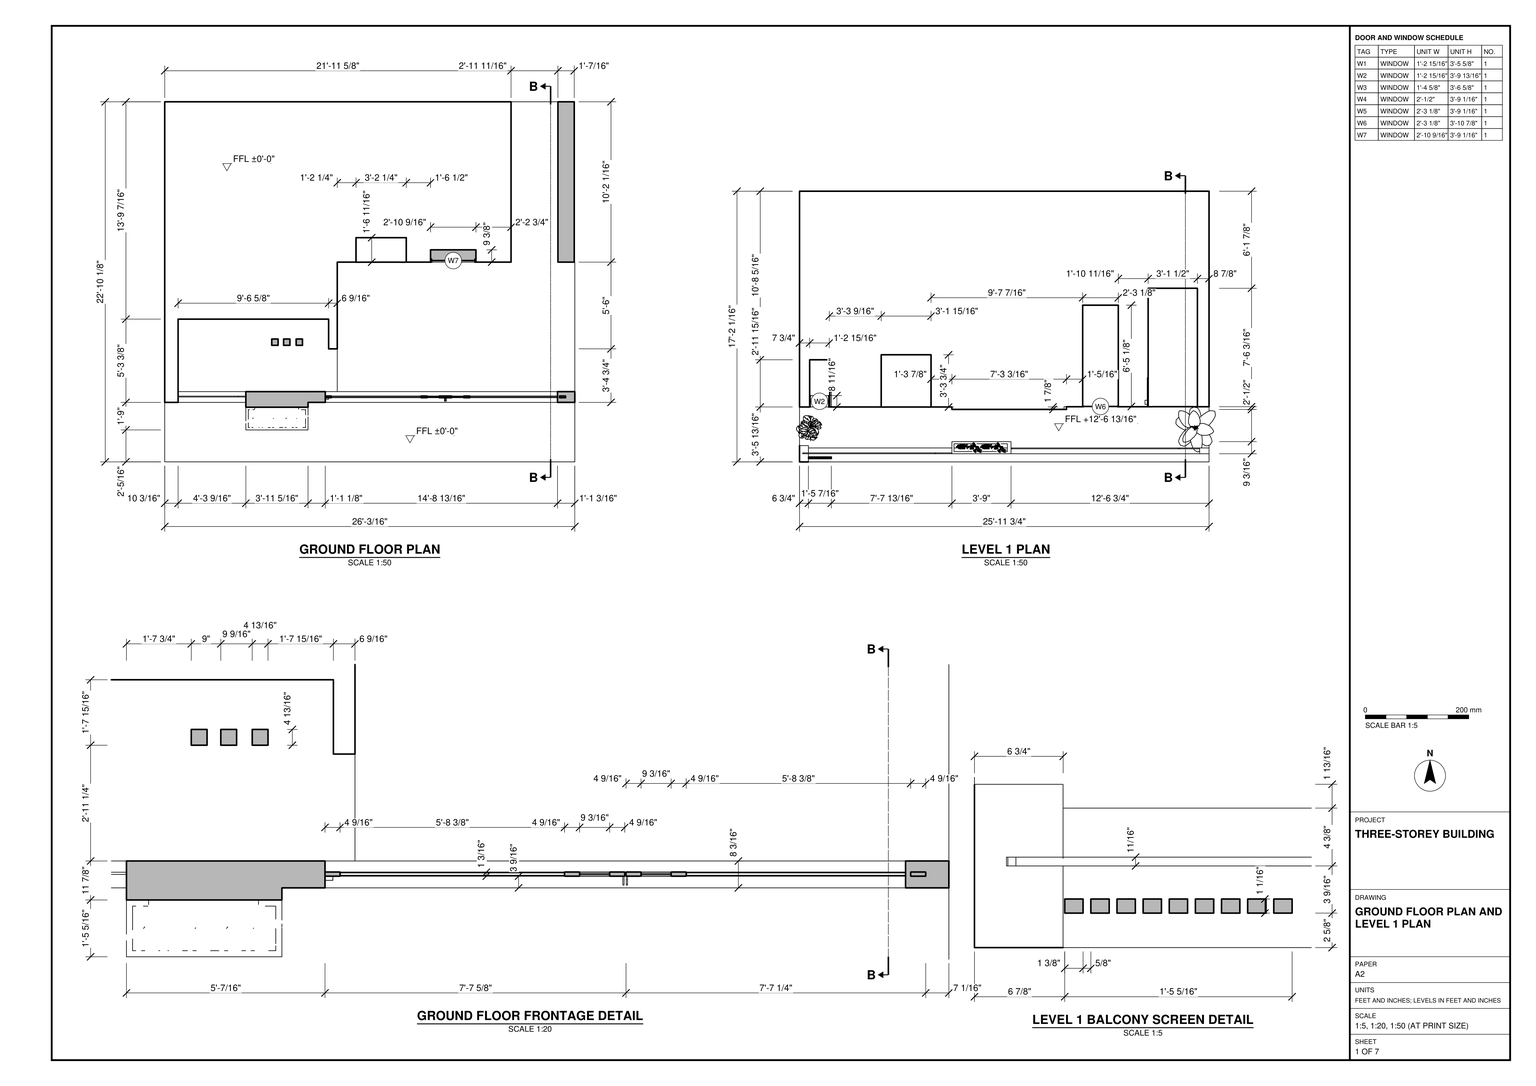
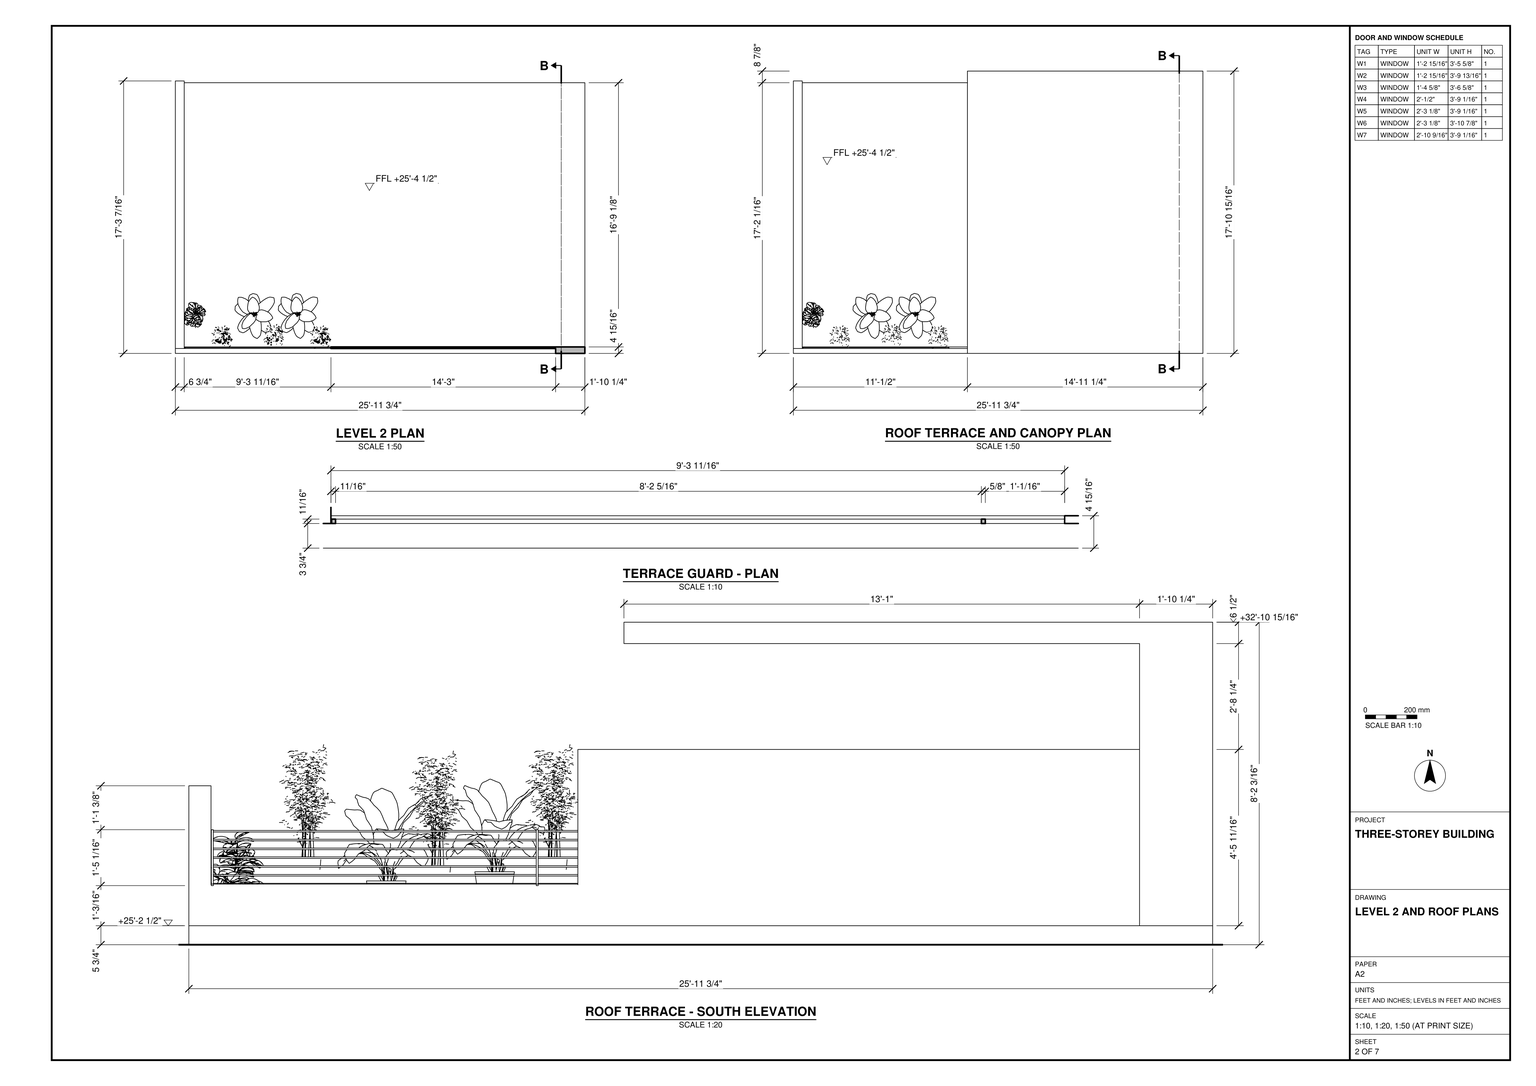
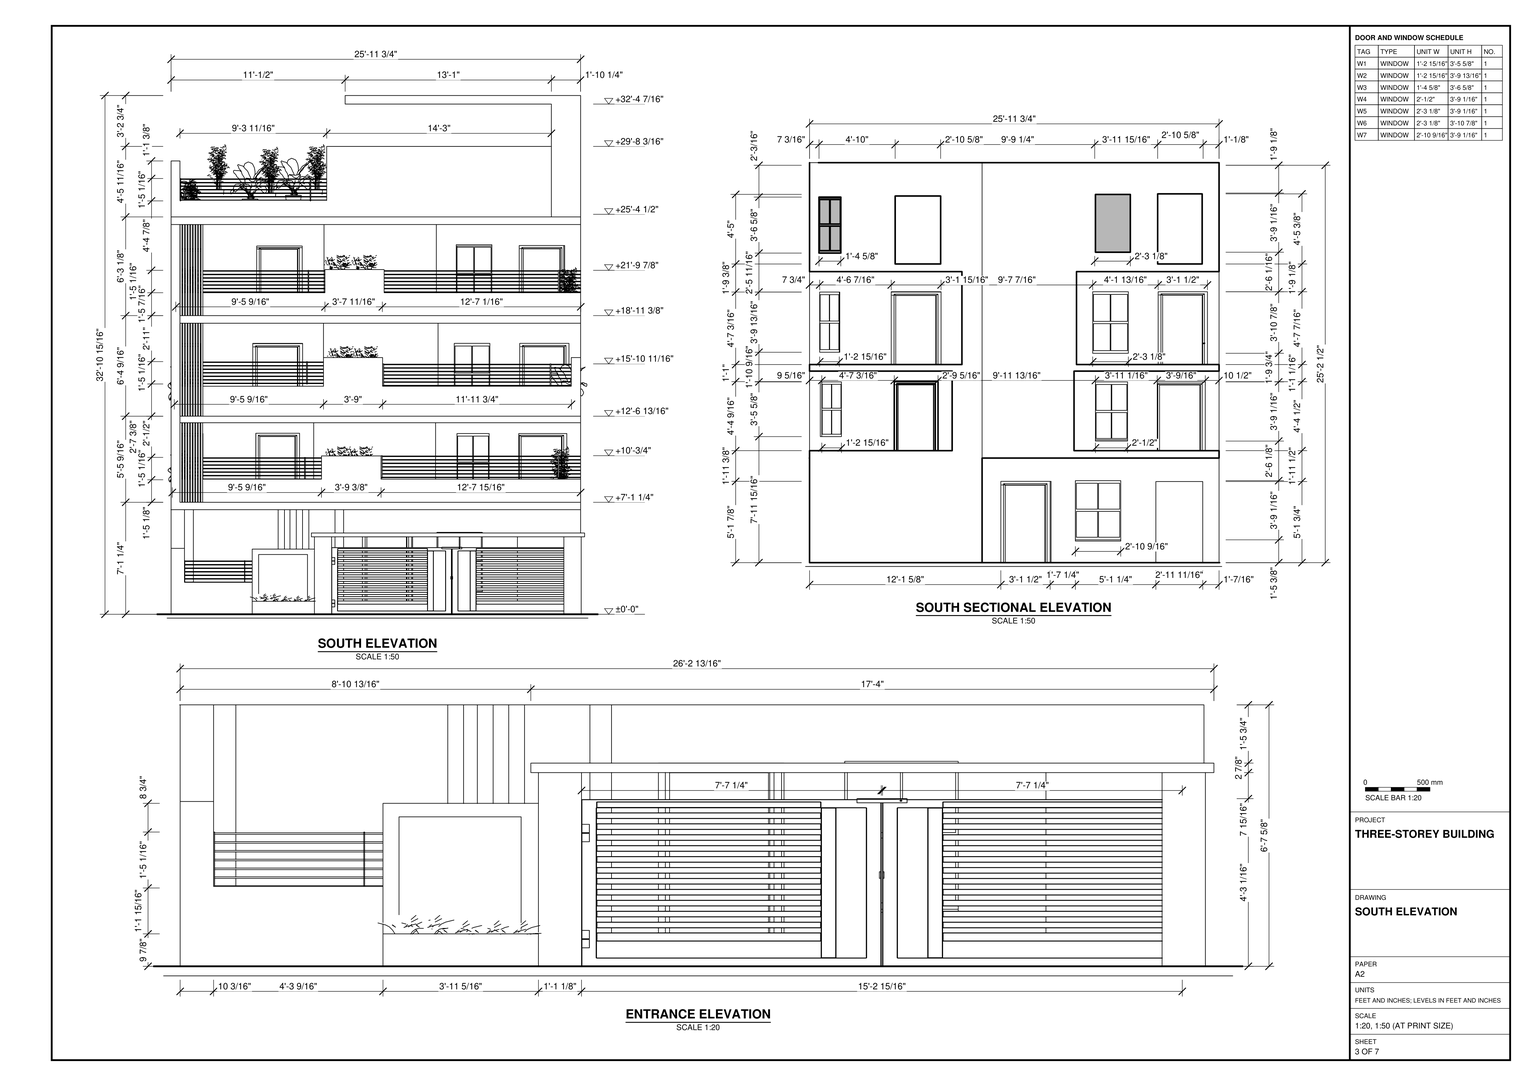
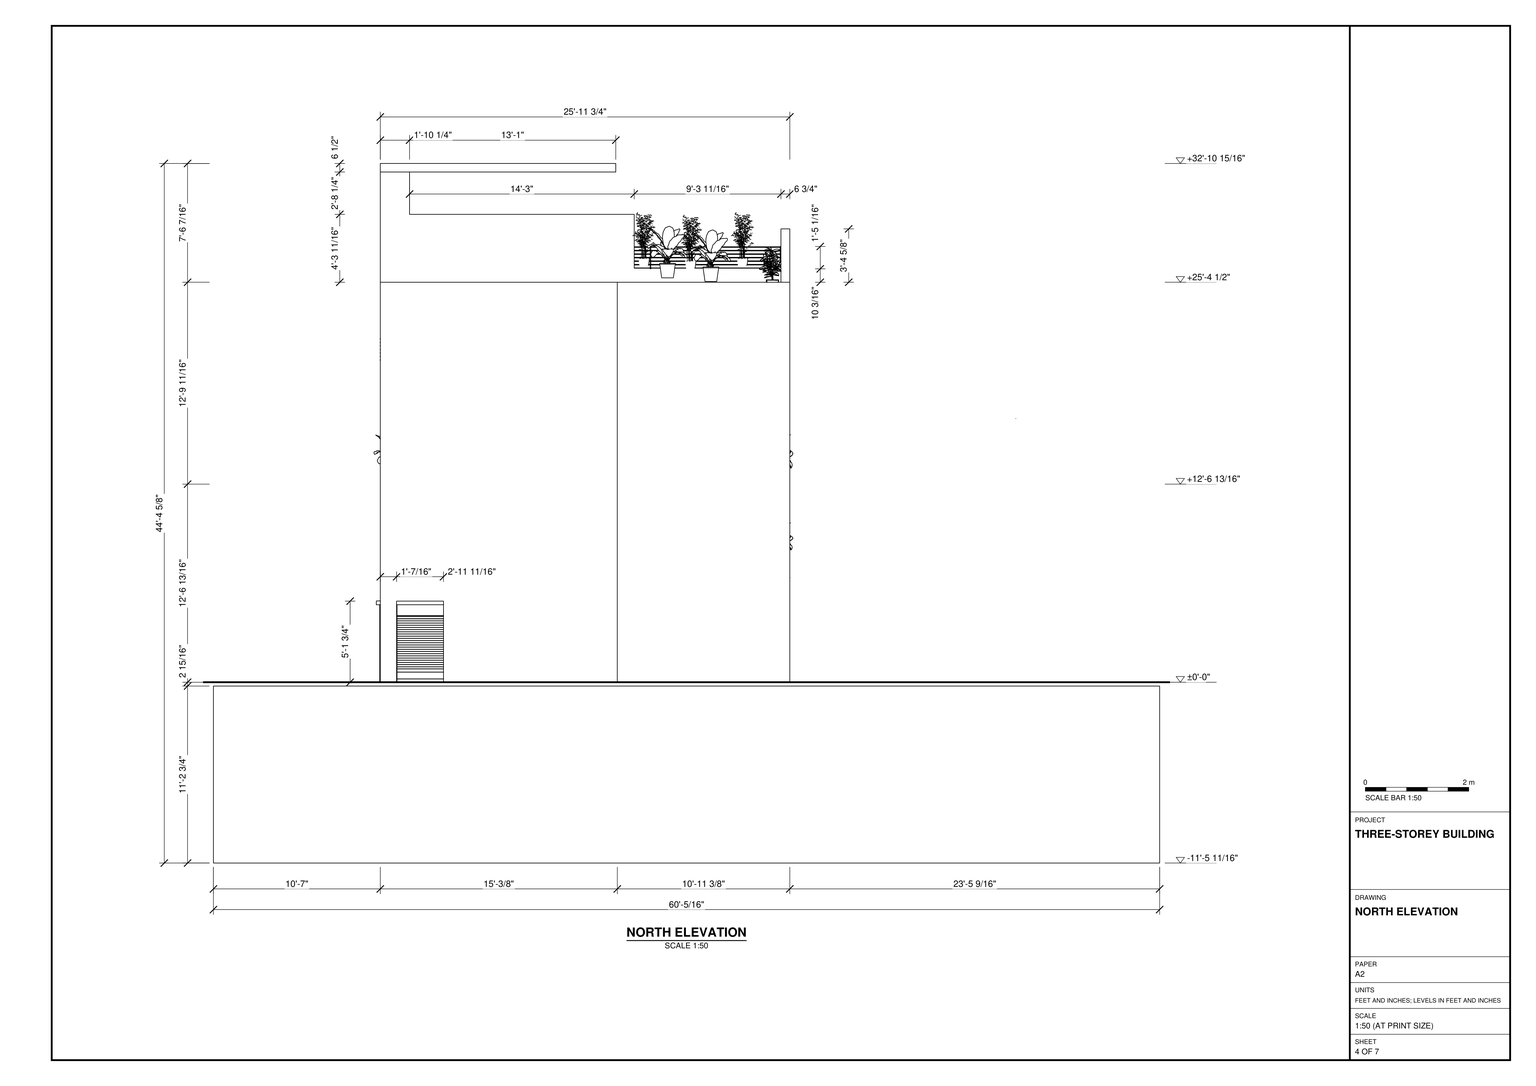
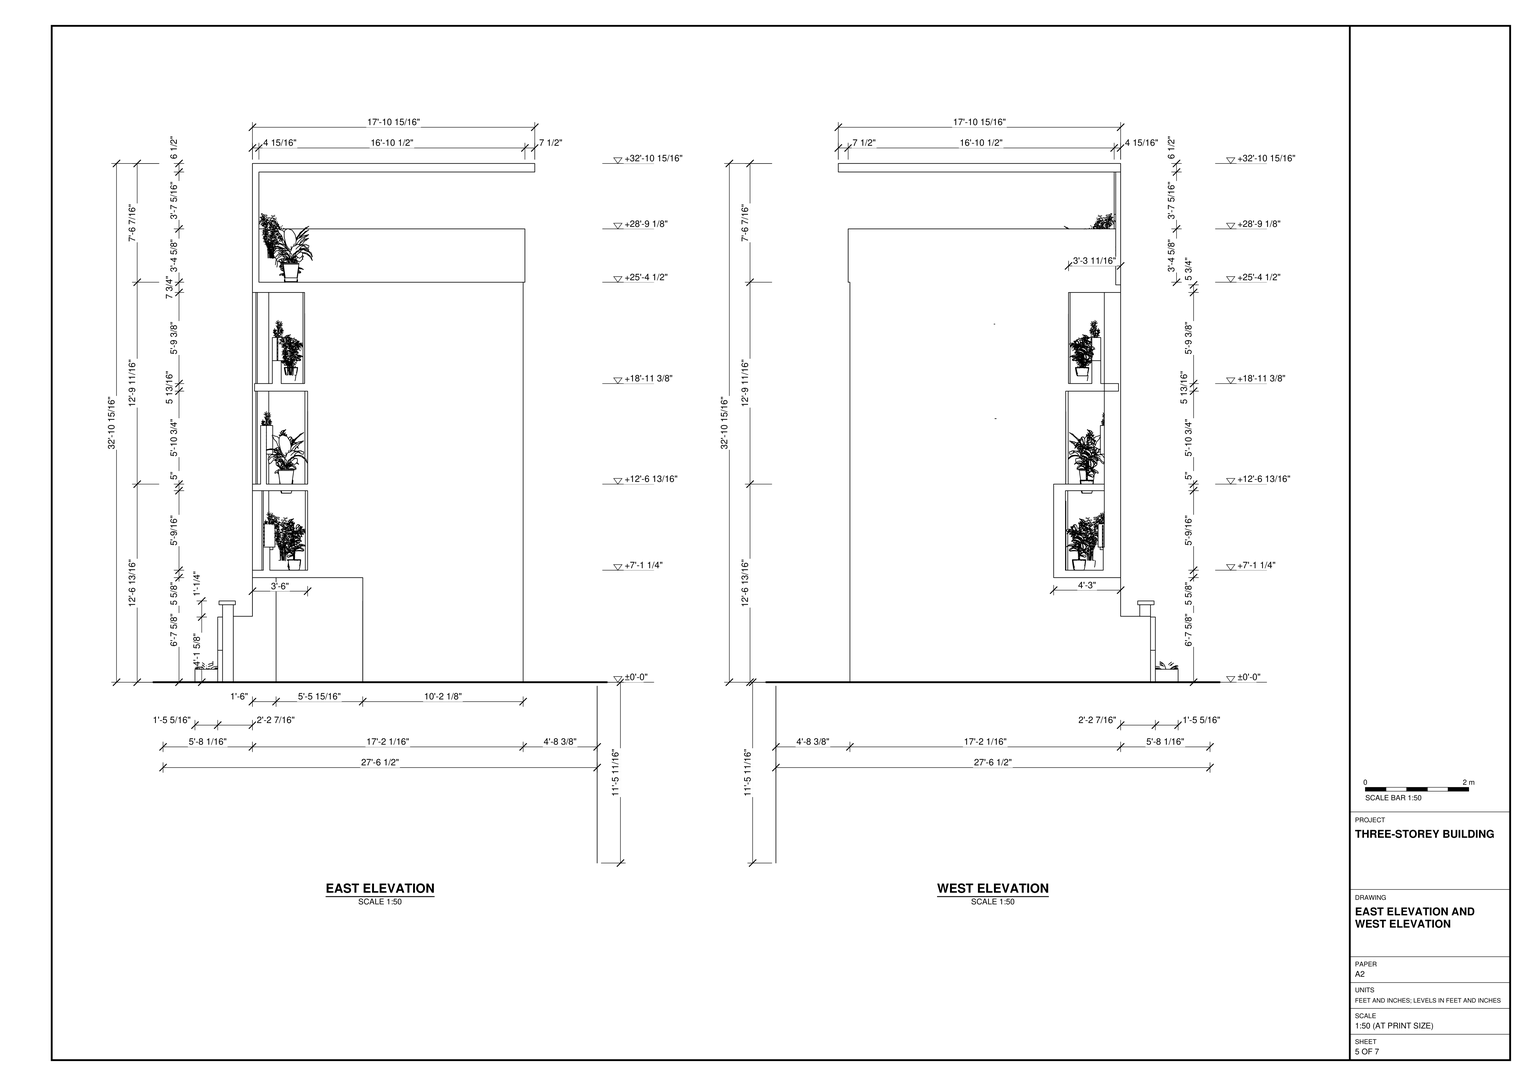
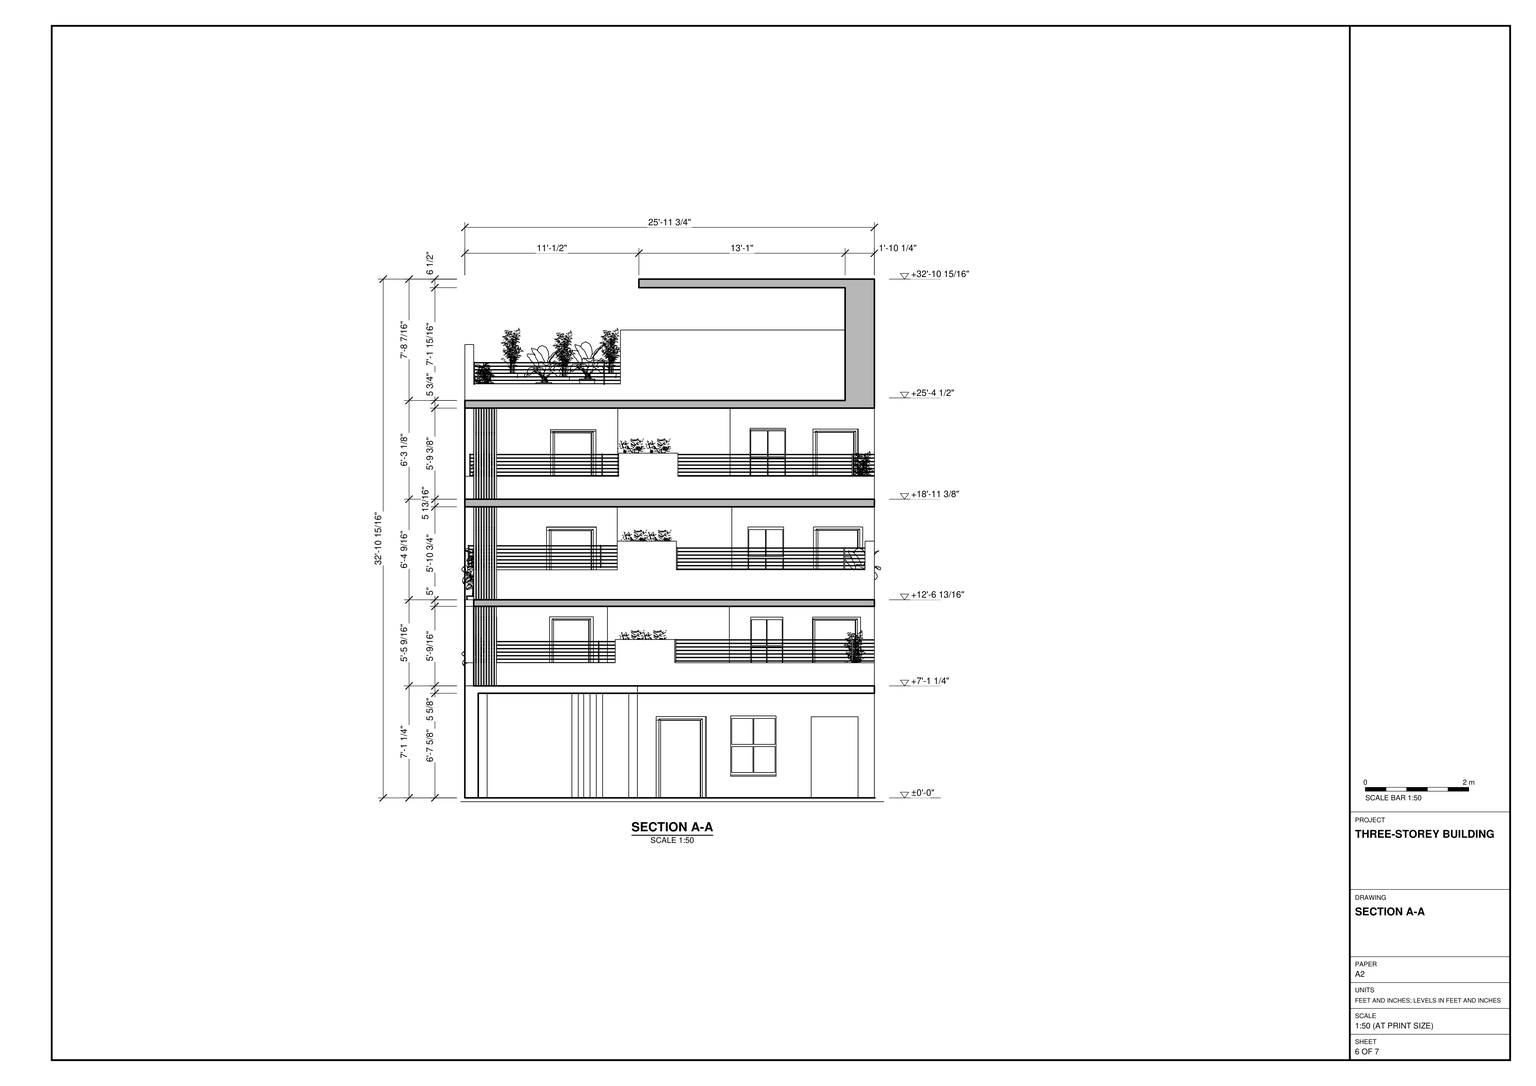
Build the three-storey building in SketchUp using task_files/diagram_01.pdf. Work in feet and inches. The complete model measures 60'-5/16" along X, 27'-6 1/2" along Y and 44'-4 5/8" along Z. Set the ground floor at ±0'-0", Level 1 at +12'-6 13/16" and Level 2 at +25'-4 1/2".

Follow the plans for the stepped ground-floor outline, wall thicknesses, upper slabs and balcony projections. Use the window schedule to size the seven window units and the south sectional elevation to position them relative to the door openings. Model the entrance with paired horizontal-slat gates beneath a projecting canopy. To their left, include the framed recess above the built-in planter and the adjoining low screen.

On the south balconies, model the horizontal guard rails, the raised planter fronts that interrupt them and the narrow vertical fins at the left end. On the roof terrace, place the guard in the opening in the left parapet and the flat canopy over the right side. Decor and loose items, including plants, may be any suitable library components placed as shown.

Keep the walls, slabs and roof elements, and each furniture or joinery piece, in separate groups or components. Use components for repeated parts. Save one SketchUp model as output_files/building_with_screened_balconies_and_roof_terrace.skp.

# SketchUp Ruby script. Lengths in inches.
U = 1.inch
M = Sketchup.active_model
def pt(a) = Geom::Point3d.new(a.map { |v| v * U })
def face(e, loops, mat)
  f = e.add_face(loops[0].map { |a| pt(a) })
  loops[1..].each { |l| e.add_face(l.map { |a| pt(a) }).erase! }
  f.material = f.back_material = mat if mat
  f
end
# faces: each face lists its corners as indices into pts; further lists are holes
def faces(e, pts, list, mat = nil) = list.each { |f| face(e, (f[0].is_a?(Array) ? f : [f]).map { |l| l.map { |i| pts[i] } }, mat) }
# xy, xz, yz: faces in a plane at the given z, y or x. An outline is a flat list of corners, or four numbers for a rectangle; further outlines are holes
def ring(l) = l.size == 4 ? [[l[0], l[1]], [l[2], l[1]], [l[2], l[3]], [l[0], l[3]]] : l.each_slice(2).to_a
def flat(e, list, mat, &to3) = list.each { |f| face(e, (f[0].is_a?(Array) ? f : [f]).map { |l| ring(l).map { |u, v| to3.(u, v) } }, mat) }
def xy(e, z, list, mat = nil) = flat(e, list, mat) { |x, y| [x, y, z] }
def xz(e, y, list, mat = nil) = flat(e, list, mat) { |x, z| [x, y, z] }
def yz(e, x, list, mat = nil) = flat(e, list, mat) { |y, z| [x, y, z] }
def lines(e, pts, list) = list.each { |a, b| e.add_line(pt(pts[a]), pt(pts[b])) }
# prism: a flat outline (further loops are holes) pulled along v
def prism(e, loops, v, mat = nil)
  f = face(e, loops, mat); d = Geom::Vector3d.new(v.map { |x| x * U })
  f.pushpull(f.normal.samedirection?(d) ? d.length : -d.length)
end
def box(e, o, s, mat = nil) = prism(e, [[o, [o[0] + s[0], o[1], o[2]], [o[0] + s[0], o[1] + s[1], o[2]], [o[0], o[1] + s[1], o[2]]]], [0, 0, s[2]], mat)
def at(x, y, z, deg = 0) = Geom::Transformation.translation(pt([x, y, z])) * Geom::Transformation.rotation(ORIGIN, Z_AXIS, deg.degrees)
def axes(o, x, y, z) = Geom::Transformation.new([*x, 0, *y, 0, *z, 0, *pt(o).to_a, 1])
def part(name) = M.definitions.add(name)
# library, detail: a bought-in or finely detailed component or shape, given as its bounding box
def library(name, o, s) = part(name).tap { |d| box(d.entities, o, s) }
def detail(e, o, s) = box(e.add_group.entities, o, s)
def put(e, d, t, mat = nil) = e.add_instance(d, t).tap { |i| i.material = mat if mat }
def group(e, t, mat = nil) = e.add_group.tap { |g| g.transformation = t; g.material = mat if mat }.entities
root = M.entities
M.materials.add("[0009_Linen]").color = [255, 234, 188]
M.materials.add("[Brick Antique 01]").color = [147, 105, 71]
M.materials.add("[Brick Tumbled]").color = [135, 132, 132]
M.materials.add("[Cladding Stucco White]").color = [200, 200, 200]
M.materials.add("[Color C01]").color = [255, 229, 204]
M.materials.add("[Color D01]").color = [255, 242, 204]
M.materials.add("[Color M00]").color = [255, 255, 255]
M.materials.add("[Grass Dark Green]").color = [106, 157, 55]
M.materials.add("[Translucent_Glass_Sky_Reflection]").color = [126, 138, 183]
M.materials["[Translucent_Glass_Sky_Reflection]"].alpha = 0.52
M.materials.add("[Wood Floor Parquet]").color = [145, 89, 39]
M.materials.add("[Wood Lumber ButtJoined]").color = [164, 152, 112]
M.materials.add("[Wood_Cherry_Original]").color = [152, 86, 42]
M.materials.add("img008").color = [189, 141, 111]
c1 = library("Group_2",[-1.28,-0.39,0],[21.22,20.51,48.44])
c2 = part("Vertical screen batten")
box(c2.entities,[0,0,0],[1.85,1.85,112.2])
c3 = part("Slatted balcony screen")
put(c3.entities,c2,at(0,0,0))
put(c3.entities,c2,at(0,13.1875,0))
put(c3.entities,c2,at(0,18.46,0))
put(c3.entities,c2,at(0,10.55,0))
put(c3.entities,c2,at(0,2.64,0))
put(c3.entities,c2,at(0,7.91,0))
put(c3.entities,c2,at(0,5.28,0))
put(c3.entities,c2,at(0,15.83,0))
put(c3.entities,c2,at(0,21.1,0))
c4 = part("window (1)")
xy(c4.entities,0,[[-0.39,0,0.39,39.37],[-0.39,39.37,0.39,40.16],[-0.39,40.16,0.39,40.94]],"[Wood_Cherry_Original]")
xy(c4.entities,0.92,[[-0.39,0.92,0,20.08],[0,0.92,0.39,20.08],[-0.39,20.87,0,39.37],[0,20.87,0.39,40.02],[-0.39,39.37,0,40.02]],"[Wood_Cherry_Original]")
xy(c4.entities,10.24,[[-0.39,0.92,0,20.08],[0,0.92,0.39,20.08],[-0.39,20.87,0,40.02],[0,20.87,0.39,40.02]],"[Wood_Cherry_Original]")
xy(c4.entities,11.02,[[-0.39,0.92,0,20.08],[0,0.92,0.39,20.08],[-0.39,20.87,0,40.02],[0,20.87,0.39,40.02]],"[Wood_Cherry_Original]")
xy(c4.entities,20.34,[[-0.39,0.92,0,20.08],[0,0.92,0.39,20.08],[-0.39,20.87,0,40.02],[0,20.87,0.39,40.02]],"[Wood_Cherry_Original]")
xy(c4.entities,21.26,[[-0.39,0,0.39,40.94]],"[Wood_Cherry_Original]")
xz(c4.entities,0,[[-0.39,0,0.39,21.26]],"[Wood_Cherry_Original]")
xz(c4.entities,0.92,[[-0.39,0.92,0,10.24],[0,0.92,0.39,10.24],[-0.39,11.02,0,20.34],[0,11.02,0.39,20.34]],"[Wood_Cherry_Original]")
xz(c4.entities,20.08,[[-0.39,0.92,0,10.24],[0,0.92,0.39,10.24],[-0.39,11.02,0,20.34],[0,11.02,0.39,20.34]],"[Wood_Cherry_Original]")
xz(c4.entities,20.87,[[-0.39,0.92,0,10.24],[0,0.92,0.39,10.24],[-0.39,11.02,0,20.34],[0,11.02,0.39,20.34]],"[Wood_Cherry_Original]")
xz(c4.entities,40.02,[[-0.39,0.92,0,10.24],[0,0.92,0.39,10.24],[-0.39,11.02,0,20.34],[0,11.02,0.39,20.34]],"[Wood_Cherry_Original]")
xz(c4.entities,40.94,[[-0.39,0,0.39,21.26]],"[Wood_Cherry_Original]")
yz(c4.entities,-0.39,[[[0,0,40.94,21.26],[20.87,0.92,40.02,10.24],[20.87,11.02,40.02,20.34],[0.92,11.02,20.08,20.34],[0.92,0.92,20.08,10.24]]],"[Wood_Cherry_Original]")
yz(c4.entities,0,[[0.92,0.92,20.08,10.24],[20.87,0.92,40.02,10.24],[0.92,11.02,20.08,20.34],[20.87,11.02,40.02,20.34]],"[Translucent_Glass_Sky_Reflection]")
yz(c4.entities,0.39,[[[0,0,40.94,21.26],[20.87,0.92,40.02,10.24],[20.87,11.02,40.02,20.34],[0.92,0.92,20.08,10.24],[0.92,11.02,20.08,20.34]]],"[Wood_Cherry_Original]")
# 1 loose lines left out
c5 = library("Broadleaf plant",[0,0,0],[149.19,166.1,98.1875])
c6 = library("Komponent\#126",[-0.02,-2.01,-1.1],[17.3,24.14,15.75])
c7 = library("VP+Bambus+Muriel",[8.93,-8.27,-0.04],[18.48,20.86,48.75])
c8 = library("Plant Banana",[3.49,5.74,0],[38.27,39.55,56.51])
c9 = part("Group\#1")
xy(c9.entities,0,[[0,0,2.125,0,2.27,0.02,2.55,0.1,2.68,0.17,2.8,0.24,2.92,0.32,3.03,0.42,3.13,0.52,3.22,0.63,3.3,0.75,3.37,0.88,3.43,1.02,3.43,1.46,0,1.46]])
xy(c9.entities,77.52,[[0.55,1.02,3.43,1.46],[3.43,1.02,34.09,1.46]])
xy(c9.entities,81.14,[[0,0,37.72,1.46]],"img008")
xz(c9.entities,0,[[0,0,0,81.14,37.72,81.14,37.72,0,35.39,0,35.39,78.82,2.125,78.82,2.125,0]],"img008")
xz(c9.entities,1.46,[[34.09,0,34.09,77.52,3.43,77.52,3.43,77.25,33.7,77.25,33.7,0.02]],"img008")
yz(c9.entities,0,[[0,0,1.46,81.14]])
yz(c9.entities,3.43,[[1.02,0,1.46,77.52]],"img008")
yz(c9.entities,34.09,[[1.02,0,1.46,77.52]],"img008")
yz(c9.entities,37.72,[[0,0,1.46,81.14]])
p = [[2.27,0.02,78.68],[2.27,0.02,0],[2.125,0,0],[2.125,0,78.82],[2.41,0.06,78.54],[2.41,0.06,0],
  [35.11,0.06,78.54],[35.25,0.02,78.68],[35.25,0.02,0],[35.11,0.06,0],[35.39,0,78.82],[35.39,0,0],
  [2.55,0.1,78.4],[2.55,0.1,0],[2.68,0.17,78.27],[2.68,0.17,0],[34.84,0.17,78.27],[34.97,0.1,78.4],
  [34.97,0.1,0],[34.84,0.17,0],[2.8,0.24,78.14],[2.8,0.24,0],[2.92,0.32,78.02],[2.92,0.32,0],
  [34.6,0.32,78.02],[34.72,0.24,78.14],[34.72,0.24,0],[34.6,0.32,0],[3.03,0.42,77.91],[3.03,0.42,0],
  [34.49,0.42,77.91],[34.49,0.42,0],[3.13,0.52,77.8125],[3.13,0.52,0],[34.39,0.52,77.8125],[34.39,0.52,0],
  [3.22,0.63,77.72],[3.22,0.63,0],[34.3,0.63,77.72],[34.3,0.63,0],[3.3,0.75,77.64],[3.3,0.75,0],
  [34.22,0.75,77.64],[34.22,0.75,0],[3.37,0.88,77.58],[3.37,0.88,0],[34.15,0.88,77.58],[34.15,0.88,0],
  [3.43,1.02,0.02],[3.43,1.02,0],[3.43,1.02,77.52],[3.43,1.02,77.25],[34.09,1.02,77.52],[34.09,1.02,0],
  [33.7,1.46,0.02],[33.7,1.46,77.25],[0.55,0.88,77.58],[0.55,1.02,77.52],[0.55,0.63,77.72],[0.55,0.75,77.64],
  [0.55,0.52,77.8125],[0.55,0.42,77.91],[0.55,0.32,78.02],[0.55,0.24,78.14]]
faces(c9.entities,p,[[0,1,2,3],[4,5,1,0],[6,7,8,9],[7,10,11,8],[12,13,5,4],[14,15,13,12],[16,17,18,19],[17,6,9,18],
  [20,21,15,14],[22,23,21,20],[24,25,26,27],[25,16,19,26],[28,29,23,22],[30,24,27,31],[32,33,29,28],[34,30,31,35],
  [36,37,33,32],[38,34,35,39],[40,41,37,36],[42,38,39,43],[44,45,41,40],[46,42,43,47],[48,49,45,44,50,51],[52,46,47,53],
  [51,48,54,55],[52,50,44,46],[42,40,36,38],[46,44,40,42],[38,36,32,34],[34,32,28,30],[30,28,22,24],[24,22,20,25],
  [25,20,14,16],[16,14,12,17],[17,12,4,6],[6,4,0,7],[7,0,3,10]],"img008")
faces(c9.entities,p,[[56,44,50,57],[58,36,40,59],[59,40,44,56],[60,32,36,58],[61,28,32,60],[62,22,28,61],[63,20,22,62]])
c10 = part("P1")
prism(c10.entities,[[[0.29,0.77,0],[0.39,0.79,0],[0.5,0.77,0],[0.59,0.73,0],[0.67,0.67,0],[0.73,0.59,0],[0.77,0.5,0],[0.79,0.39,0],[0.77,0.29,0],[0.73,0.2,0],[0.67,0.12,0],[0.59,0.05,0],[0.5,0.01,0],[0.39,0,0],[0.29,0.01,0],[0.2,0.05,0],[0.12,0.12,0],[0.05,0.2,0],[0.01,0.29,0],[0,0.39,0],[0.01,0.5,0],[0.05,0.59,0],[0.12,0.67,0],[0.2,0.73,0]]],[0,0,72.83])
# 1 loose lines left out
c11 = part("bareau P1\#1")
prism(c11.entities,[[[0,27.72,7.875],[0,28.5,7.875],[0.79,28.5,7.875],[0.79,0,7.875],[0,0,7.875]]],[0,0,0.39])
# 2 loose lines left out
c12 = part("Group\#2")
p = [[72.83,0.39,27.72],[72.83,0.79,27.72]]
lines(c12.entities,p,[[0,1]])
put(c12.entities,c10,axes([72.83,0,28.11],[0,1,0],[0,0,-1],[-1,0,0]),"[Wood Floor Parquet]")
put(c12.entities,c10,axes([72.83,0,19.13],[0,1,0],[0,0,-1],[-1,0,0]),"[Wood Floor Parquet]")
put(c12.entities,c10,axes([72.83,0,14.65],[0,1,0],[0,0,-1],[-1,0,0]),"[Wood Floor Parquet]")
put(c12.entities,c10,axes([72.83,0,10.16],[0,1,0],[0,0,-1],[-1,0,0]),"[Wood Floor Parquet]")
put(c12.entities,c10,axes([72.83,0,5.67],[0,1,0],[0,0,-1],[-1,0,0]),"[Wood Floor Parquet]")
put(c12.entities,c10,axes([72.83,0,1.18],[0,1,0],[0,0,-1],[-1,0,0]),"[Wood Floor Parquet]")
put(c12.entities,c11,axes([72.83,0,28.5],[0,1,0],[0,0,-1],[-1,0,0]),"[Wood Floor Parquet]")
put(c12.entities,c10,axes([72.83,0,23.62],[0,1,0],[0,0,-1],[-1,0,0]),"[Wood Floor Parquet]")
put(c12.entities,c11,axes([8.33,0,28.5],[0,1,0],[0,0,-1],[-1,0,0]),"[Wood Floor Parquet]")
c13 = library("Group\#4",[0,0,0],[107.6,5.33,60.06])
xy(root,0,[[345.16,26.17,388.76,26.17,388.76,39.74,383.49,39.74,383.49,43.42,350.05,43.42,350.05,39.74,345.16,39.74],[343.29,41.6,348.18,41.6,348.18,45.29,385.36,45.29,385.36,41.6,390.63,41.6,390.63,45.29,403.75,45.29,403.75,53.48,291.71,53.48,291.71,108.67,406.31,108.67,406.31,86.04,412.88,86.04,412.88,152.06,427.16,152.06,427.16,170.68,465.41,170.68,465.41,152.06,545.17,152.06,545.17,274.125,281.53,274.125,281.53,45.29,343.29,45.29],[403.75,45.29,580.53,53.48],[580.53,45.29,593.72,53.48],[[291.71,53.48,412.88,53.48,412.88,86.04,406.31,86.04,406.31,108.67,291.71,108.67],[363.02,88.73,367.84,93.54],[372.02,88.73,376.84,93.54],[381.59,88.73,386.4,93.54]],
  [363.02,88.73,367.84,93.54],[372.02,88.73,376.84,93.54],[381.59,88.73,386.4,93.54],[580.86,152.06,593.28,274.125]])
xy(root,0,[[281.53,0,593.72,0,593.72,45.29,390.63,45.29,390.63,24.3,343.29,24.3,343.29,45.29,281.53,45.29]],"[Brick Tumbled]")
xy(root,0,[[412.88,53.48,593.72,53.48,593.72,152.06,580.86,152.06,580.86,274.125,545.17,274.125,545.17,152.06,465.41,152.06,465.41,170.68,427.16,170.68,427.16,152.06,412.88,152.06]],"[Cladding Stucco White]")
xy(root,9.875,[[[343.29,24.3,390.63,24.3,390.63,41.6,385.36,41.6,385.36,45.29,348.18,45.29,348.18,41.6,343.29,41.6],[345.16,26.17,345.16,39.74,350.05,39.74,350.05,43.42,383.49,43.42,383.49,39.74,388.76,39.74,388.76,26.17]]],"[Brick Tumbled]")
xy(root,16.41,[[483.89,152.06,518.45,161.43]])
xy(root,24.3125,[[291.71,45.29,343.29,53.48]])
xy(root,45.51,[[348.18,41.6,385.36,45.29]])
xy(root,49.625,[[343.29,41.6,390.63,53.48]])
xy(root,50.1875,[[281.53,45.29,291.71,68.04]])
xy(root,58.98,[[390.63,45.29,403.75,53.48]])
xy(root,58.98,[[388.32,42.6,390.63,55.04],[403.75,45.29,596.3125,55.04],[390.63,53.48,403.75,55.04]],"[Brick Tumbled]")
xy(root,58.98,[[390.63,42.6,596.3125,45.29]],"[Color M00]")
xy(root,59.1875,[[580.53,45.29,593.72,53.48]])
xy(root,61.75,[[545.17,152.06,580.86,274.125]])
xy(root,61.88,[[388.32,42.6,596.3125,55.04]],"[Brick Tumbled]")
xy(root,61.89,[[427.16,152.06,465.41,170.68]])
xy(root,62.41,[[483.89,152.06,518.45,161.43]])
xy(root,79.625,[[291.71,68.04,298.49,108.67],[298.49,68.04,298.49,108.67,374.98,108.67,374.98,93.54,372.02,93.54,372.02,88.73,374.98,88.73,374.98,68.04],[374.98,68.04,374.98,88.73,376.84,88.73,376.84,93.54,374.98,93.54,374.98,108.67,406.31,108.67,406.31,68.04],[406.31,68.04,412.88,86.04],[412.88,68.04,593.28,152.06],
  [363.02,88.73,367.84,93.54],[372.02,88.73,374.98,93.54],[374.98,88.73,376.84,93.54],[381.59,88.73,386.4,93.54],[281.33,108.67,281.53,119.05]])
xy(root,85.25,[[288.28,68.04,593.28,76.35],[281.53,81.29,593.28,81.29,593.28,110.05,582.77,110.05,582.77,132.24,546.21,132.24,546.21,110.05,482.88,110.05,482.88,108.3,390.09,108.3,390.09,110.05,379.34,110.05,379.34,129.11,346.09,129.11,346.09,110.05,281.53,110.05]])
xy(root,93.48,[[499.15,110.05,523.65,137.42]])
xy(root,95.95,[[289.72,110.05,305.78,121.55]])
xy(root,100.9375,[[397.54,77.875,439.83,83.64]])
xy(root,102.875,[[288.28,76.35,396.01,76.35,396.01,81.29,281.53,81.29,281.53,80.47,288.28,80.47],[441.36,76.35,593.28,81.29],[396.01,81.29,441.36,85.17]])
xy(root,120.5625,[[[396.01,76.35,441.36,85.17],[397.54,77.875,439.83,83.64]]])
xy(root,137.6,[[289.72,110.05,305.78,121.55],[346.09,110.05,379.34,129.11],[499.15,110.05,523.65,137.42],[546.21,110.05,582.77,132.24]])
xy(root,145.8125,[[288.28,68.04,288.28,80.47,281.53,80.47,281.53,110.05,390.09,110.05,390.09,68.04],[482.88,68.04,593.28,110.05]])
xy(root,145.8125,[[390.09,68.04,482.88,108.3]],"[Wood Lumber ButtJoined]")
xy(root,150.8125,[[288.28,68.04,593.28,74.26],[288.28,78.66,593.28,78.66,593.28,110.05,584.43,110.05,584.43,200.24,546.92,200.24,546.92,110.05,484.76,110.05,484.76,107.99,397.54,107.99,397.54,109.86,381.66,109.86,381.66,149.61,343.72,149.61,343.72,109.86,281.53,109.86,281.53,80.47,288.28,80.47]])
xy(root,159.375,[[497.08,110.05,524.21,187.36]])
xy(root,160.1875,[[289.25,109.86,304.57,145.8]])
xy(root,173.625,[[288.28,74.26,397.54,78.66],[442.54,74.26,586.16,78.66],[399.15,75.86,439.74,78.66],[397.54,78.66,397.54,83.47,442.54,83.47,442.54,78.66,439.74,78.66,439.74,81.86,399.15,81.86,399.15,78.66],[399.15,78.66,439.74,81.86]])
xy(root,195.4375,[[[397.54,74.26,442.54,83.47],[399.15,75.86,439.74,81.86]],[586.16,74.26,593.28,78.66]])
xy(root,206,[[289.25,109.86,304.57,145.8]])
xy(root,206.25,[[343.72,109.86,381.66,149.61],[497.08,110.05,524.21,187.36],[546.92,110.05,584.43,200.24]])
xy(root,221.57,[[281.53,69.67,397.54,109.86],[397.54,69.67,484.76,107.99],[484.76,69.67,593.28,110.05]])
xy(root,227.375,[[281.53,69.67,593.28,83.2],[281.53,89.94,593.28,89.94,593.28,107.71,580.41,107.71,580.41,154.83,546.54,154.83,546.54,107.71,483.45,107.71,483.45,106.52,397.95,106.52,397.95,107.71,381.33,107.71,381.33,132.71,346.71,132.71,346.71,107.71,281.53,107.71]])
xy(root,235.66,[[288.73,107.71,305.35,127.83]])
xy(root,236.31,[[499.17,107.71,525.73,125.14]])
xy(root,244.8125,[[281.53,83.2,398.66,89.94],[443.72,83.2,593.28,89.94],[398.66,89.94,443.72,93.51]])
xy(root,260.3125,[[399.44,87.86,442.9375,92.72]])
xy(root,262.4375,[[[398.66,83.2,443.72,93.51],[399.44,87.86,442.9375,92.72]]])
xy(root,277.85,[[288.73,107.71,305.35,127.83]])
xy(root,279.125,[[346.71,107.71,381.33,132.71]])
xy(root,280.31,[[499.17,107.71,525.73,125.14]])
xy(root,280.75,[[546.54,107.71,580.41,154.83]])
xy(root,296.73,[[281.53,68.04,397.95,107.71],[397.95,68.04,483.45,106.52],[483.45,68.04,593.28,107.71]])
xy(root,302.51,[[281.53,68.04,571.02,71.79]])
xy(root,304.5,[[288.28,72.97,593.28,274.125],[281.53,274.125,288.28,275.47]])
xy(root,315.1875,[[288.28,71.79,399.99,72.97]])
xy(root,345.125,[[281.53,71.79,288.28,275.47]])
xy(root,356.1875,[[399.99,71.79,571.02,72.97]])
xy(root,388.43,[[414.02,68.04,414.02,282.97,593.28,282.97,593.28,72.97,571.02,72.97,571.02,68.04]],"[Color D01]")
xy(root,394.9375,[[414.02,68.04,593.28,282.97]])
xz(root,24.3,[[343.29,0,390.63,9.875]],"[Brick Tumbled]")
xz(root,26.17,[[345.16,0,388.76,9.875]])
xz(root,39.74,[[345.16,0,350.05,9.875],[383.49,0,388.76,9.875]])
xz(root,41.6,[[343.29,0,348.18,9.875],[385.36,0,390.63,9.875],[343.29,9.875,348.18,9.875,348.18,45.51,385.36,45.51,385.36,9.875,390.63,9.875,390.63,49.625,343.29,49.625]])
xz(root,42.6,[[388.32,58.98,596.3125,61.88]],"[Brick Tumbled]")
xz(root,43.42,[[350.05,0,383.49,9.875]])
xz(root,45.29,[[348.18,0,385.36,9.875]])
xz(root,45.29,[[390.63,0,403.75,58.98],[580.53,0,593.72,58.98],[580.53,58.98,593.72,59.1875]],"[Brick Tumbled]")
xz(root,45.29,[[281.53,0,343.29,0,343.29,24.3125,291.71,24.3125,291.71,50.1875,281.53,50.1875]],"[Color C01]")
xz(root,53.48,[[580.53,0,593.72,59.1875]])
xz(root,53.48,[[291.71,0,291.71,24.3125,343.29,24.3125,343.29,49.625,390.63,49.625,390.63,58.98,403.75,58.98,403.75,0]],"[Brick Tumbled]")
xz(root,55.04,[[388.32,58.98,596.3125,61.88]],"[Brick Tumbled]")
xz(root,68.04,[[281.53,50.1875,291.71,79.625]])
xz(root,68.04,[[281.53,79.625,593.28,79.625,593.28,85.25,288.28,85.25,288.28,296.73,281.53,296.73],[288.28,145.8125,593.28,150.8125],[571.02,302.51,593.28,302.51,593.28,394.9375,414.02,394.9375,414.02,388.43,571.02,388.43]],"[Color C01]")
xz(root,68.04,[[281.53,296.73,593.28,302.51]],"[Color D01]")
xz(root,69.67,[[281.53,221.57,593.28,227.375]],"[Color C01]")
xz(root,71.79,[[281.53,302.51,571.02,302.51,571.02,356.1875,399.99,356.1875,399.99,315.1875,288.28,315.1875,288.28,345.125,281.53,345.125]],"[Color C01]")
xz(root,72.97,[[288.28,304.5,288.28,315.1875,399.99,315.1875,399.99,356.1875,571.02,356.1875,571.02,388.43,593.28,388.43,593.28,304.5]])
xz(root,74.26,[[288.28,150.8125,593.28,150.8125,593.28,195.4375,586.16,195.4375,586.16,173.625,442.54,173.625,442.54,195.4375,397.54,195.4375,397.54,173.625,288.28,173.625]],"[Color D01]")
xz(root,75.86,[[399.15,173.625,439.74,195.4375]])
xz(root,76.35,[[288.28,85.25,593.28,85.25,593.28,102.875,441.36,102.875,441.36,120.5625,396.01,120.5625,396.01,102.875,288.28,102.875]],"[Color C01]")
xz(root,77.875,[[397.54,100.9375,439.83,120.5625]])
xz(root,78.66,[[288.28,150.8125,586.16,173.625],[586.16,150.8125,593.28,195.4375]])
xz(root,80.47,[[281.53,102.875,288.28,145.8125],[281.53,145.8125,288.28,150.8125]])
xz(root,81.29,[[281.53,85.25,593.28,102.875]])
xz(root,81.86,[[399.15,173.625,439.74,195.4375]])
xz(root,83.2,[[281.53,227.375,593.28,227.375,593.28,244.8125,443.72,244.8125,443.72,262.4375,398.66,262.4375,398.66,244.8125,281.53,244.8125]],"[Color D01]")
xz(root,83.47,[[397.54,173.625,442.54,195.4375]])
xz(root,83.64,[[397.54,100.9375,439.83,120.5625]])
xz(root,85.17,[[396.01,102.875,441.36,120.5625]])
xz(root,86.04,[[406.31,0,412.88,79.625]],"[Color C01]")
xz(root,87.86,[[399.44,260.3125,442.9375,262.4375]])
xz(root,88.73,[[363.02,0,367.84,79.625],[372.02,0,376.84,79.625],[381.59,0,386.4,79.625]],"[Wood Floor Parquet]")
xz(root,89.94,[[281.53,227.375,593.28,244.8125]])
xz(root,92.72,[[399.44,260.3125,442.9375,262.4375]])
xz(root,93.51,[[398.66,244.8125,443.72,262.4375]])
xz(root,93.54,[[363.02,0,367.84,71.625],[372.02,0,376.84,79.625],[381.59,0,386.4,1.6875],[381.59,1.6875,386.4,79.625],[363.02,71.625,367.84,79.625]])
xz(root,106.52,[[397.95,227.375,483.45,296.73]],"[Wood Lumber ButtJoined]")
xz(root,107.71,[[[281.53,227.375,346.71,227.375,346.71,279.125,381.33,279.125,381.33,227.375,397.95,227.375,397.95,296.73,281.53,296.73],[288.73,235.66,305.35,277.85]]],"[Color C01]")
xz(root,107.71,[[[483.45,227.375,546.54,227.375,546.54,280.75,580.41,280.75,580.41,227.375,593.28,227.375,593.28,296.73,483.45,296.73],[499.17,236.31,525.73,280.31]]],"[Color D01]")
xz(root,107.99,[[397.54,150.8125,484.76,221.57]],"[Wood Lumber ButtJoined]")
xz(root,108.3,[[390.09,85.25,482.88,145.8125]],"[Wood Lumber ButtJoined]")
xz(root,108.67,[[298.49,0,374.98,79.625]],"[Brick Antique 01]")
xz(root,108.67,[[374.98,0,406.31,79.625]],"[Color C01]")
xz(root,108.67,[[291.71,0,298.49,79.625]],"[Color D01]")
xz(root,109.86,[[[281.53,150.8125,343.72,150.8125,343.72,206.25,381.66,206.25,381.66,150.8125,397.54,150.8125,397.54,221.57,281.53,221.57],[289.25,160.1875,304.57,206]]],"[Color D01]")
xz(root,110.05,[[[281.53,85.25,346.09,85.25,346.09,137.6,379.34,137.6,379.34,85.25,390.09,85.25,390.09,145.8125,281.53,145.8125],[289.72,95.95,305.78,137.6]],[[482.88,85.25,546.21,85.25,546.21,137.6,582.77,137.6,582.77,85.25,593.28,85.25,593.28,145.8125,482.88,145.8125],[499.15,93.48,523.65,137.6]],[[484.76,150.8125,546.92,150.8125,546.92,206.25,584.43,206.25,584.43,150.8125,593.28,150.8125,593.28,221.57,484.76,221.57],[497.08,159.375,524.21,206.25]]],"[Color D01]")
xz(root,121.55,[[289.72,95.95,305.78,137.6]])
xz(root,125.14,[[499.17,236.31,525.73,280.31]])
xz(root,127.83,[[288.73,235.66,305.35,277.85]])
xz(root,129.11,[[346.09,85.25,379.34,137.6]])
xz(root,132.24,[[546.21,85.25,582.77,137.6]])
xz(root,132.71,[[346.71,227.375,381.33,279.125]])
xz(root,137.42,[[499.15,93.48,523.65,137.6]])
xz(root,145.8,[[289.25,160.1875,304.57,206]])
xz(root,149.61,[[343.72,150.8125,381.66,206.25]])
xz(root,152.06,[[[412.88,0,427.16,0,427.16,61.89,465.41,61.89,465.41,0,545.17,0,545.17,61.75,580.86,61.75,580.86,0,593.28,0,593.28,79.625,412.88,79.625],[483.89,16.41,518.45,62.41]]],"[Color D01]")
xz(root,154.83,[[546.54,227.375,580.41,280.75]])
xz(root,161.43,[[483.89,16.41,518.45,62.41]])
xz(root,170.68,[[427.16,0,465.41,61.89]])
xz(root,187.36,[[497.08,159.375,524.21,206.25]])
xz(root,200.24,[[546.92,150.8125,584.43,206.25]])
xz(root,274.125,[[281.53,0,412.88,304.5],[412.88,0,412.88,304.5,593.28,304.5,593.28,0,580.86,0,580.86,61.75,545.17,61.75,545.17,0]])
xz(root,275.47,[[281.53,304.5,288.28,345.125]])
xz(root,282.97,[[414.02,388.43,593.28,394.9375]])
xz(root,330.47,[[0,-137.67,720.3125,-2.92]],"[Grass Dark Green]")
yz(root,109.53,[[162.76,200.66,163.75,200.7]],"img008")
yz(root,281.53,[[45.29,0,45.29,50.1875,68.04,50.1875,68.04,79.625,119.05,79.625,119.05,150.8125,109.86,150.8125,109.86,221.57,80.47,221.57,80.47,227.375,83.2,227.375,83.2,244.8125,89.94,244.8125,89.94,227.375,107.71,227.375,107.71,296.73,68.04,296.73,68.04,302.51,71.79,302.51,71.79,345.125,275.47,345.125,275.47,304.5,274.125,304.5,274.125,0],[[68.04,79.625,68.04,296.73,80.47,296.73,80.47,150.8125,119.05,150.8125,119.05,79.625],[81.29,85.25,110.05,85.25,110.05,145.8125,80.47,145.8125,80.47,102.875,81.29,102.875]],[69.67,221.57,80.47,227.375]])
yz(root,288.28,[[68.04,85.25,76.35,85.25,76.35,102.875,80.47,102.875,80.47,145.8125,68.04,145.8125],[68.04,145.8125,80.47,145.8125,80.47,150.8125,78.66,150.8125,78.66,173.625,74.26,173.625,74.26,150.8125,68.04,150.8125],[78.66,150.8125,80.47,173.625],[71.79,315.1875,72.97,345.125]])
yz(root,288.28,[[72.97,304.5,275.47,345.125]],"[0009_Linen]")
yz(root,288.73,[[107.71,235.66,127.83,277.85]])
yz(root,289.25,[[109.86,160.1875,145.8,206]])
yz(root,289.72,[[110.05,95.95,121.55,137.6]])
yz(root,291.71,[[53.48,0,108.67,0,108.67,79.625,68.04,79.625,68.04,50.1875,45.29,50.1875,45.29,24.3125,53.48,24.3125]],"[Color C01]")
yz(root,304.57,[[109.86,160.1875,145.8,206]])
yz(root,305.35,[[107.71,235.66,127.83,277.85]])
yz(root,305.78,[[110.05,95.95,121.55,137.6]])
yz(root,343.29,[[41.6,0,45.29,24.3125]])
yz(root,343.29,[[24.3,0,41.6,9.875],[41.6,24.3125,53.48,49.625]],"[Brick Tumbled]")
yz(root,343.72,[[109.86,150.8125,149.61,206.25]])
yz(root,345.16,[[26.17,0,39.74,9.875]])
yz(root,346.09,[[110.05,85.25,129.11,137.6]])
yz(root,346.71,[[107.71,227.375,132.71,279.125]])
yz(root,348.18,[[41.6,0,45.29,9.875],[41.6,9.875,45.29,45.51]])
yz(root,350.05,[[39.74,0,43.42,9.875]])
yz(root,363.02,[[88.73,71.625,93.54,79.625]])
yz(root,363.02,[[88.73,0,93.54,71.625]],"[Wood Floor Parquet]")
yz(root,367.84,[[88.73,71.625,93.54,79.625]])
yz(root,367.84,[[88.73,0,93.54,71.625]],"[Wood Floor Parquet]")
yz(root,372.02,[[88.73,0,93.54,79.625]],"[Wood Floor Parquet]")
yz(root,376.84,[[88.73,0,93.54,79.625]],"[Wood Floor Parquet]")
yz(root,379.34,[[110.05,85.25,129.11,137.6]])
yz(root,381.33,[[107.71,227.375,132.71,279.125]])
yz(root,381.59,[[88.73,0,93.54,1.6875]])
yz(root,381.59,[[88.73,1.6875,93.54,79.625]],"[Wood Floor Parquet]")
yz(root,381.66,[[109.86,150.8125,149.61,206.25]])
yz(root,383.49,[[39.74,0,43.42,9.875]])
yz(root,385.36,[[41.6,0,45.29,9.875],[41.6,9.875,45.29,45.51]])
yz(root,386.4,[[88.73,0,93.54,1.6875]])
yz(root,386.4,[[88.73,1.6875,93.54,79.625]],"[Wood Floor Parquet]")
yz(root,388.32,[[42.6,58.98,55.04,61.88]],"[Brick Tumbled]")
yz(root,388.76,[[26.17,0,39.74,9.875]])
yz(root,390.09,[[108.3,85.25,110.05,145.8125]])
yz(root,390.63,[[41.6,0,45.29,24.3125],[41.6,24.3125,45.29,49.625]])
yz(root,390.63,[[24.3,0,41.6,9.875],[45.29,49.625,53.48,58.98]],"[Brick Tumbled]")
yz(root,396.01,[[76.35,102.875,85.17,120.5625]])
yz(root,397.54,[[77.875,100.9375,83.64,120.5625],[107.99,150.8125,109.86,221.57],[74.26,173.625,83.47,195.4375]])
yz(root,397.95,[[106.52,227.375,107.71,296.73]])
yz(root,398.66,[[83.2,244.8125,93.51,262.4375]])
yz(root,399.15,[[75.86,173.625,81.86,195.4375]])
yz(root,399.44,[[87.86,260.3125,92.72,262.4375]])
yz(root,399.99,[[71.79,315.1875,72.97,356.1875]])
yz(root,403.75,[[45.29,0,53.48,58.98]],"[Brick Tumbled]")
yz(root,406.31,[[86.04,0,108.67,79.625]])
yz(root,412.88,[[86.04,0,152.06,79.625]])
yz(root,414.02,[[68.04,388.43,282.97,394.9375]])
yz(root,427.16,[[152.06,0,170.68,61.89]])
yz(root,439.74,[[75.86,173.625,81.86,195.4375]])
yz(root,439.83,[[77.875,100.9375,83.64,120.5625]])
yz(root,441.36,[[76.35,102.875,85.17,120.5625]])
yz(root,442.54,[[74.26,173.625,83.47,195.4375]])
yz(root,442.9375,[[87.86,260.3125,92.72,262.4375]])
yz(root,443.72,[[83.2,244.8125,93.51,262.4375]])
yz(root,465.41,[[152.06,0,170.68,61.89]])
yz(root,482.88,[[108.3,85.25,110.05,145.8125]])
yz(root,483.45,[[106.52,227.375,107.71,296.73]])
yz(root,483.89,[[152.06,16.41,161.43,62.41]])
yz(root,484.76,[[107.99,150.8125,110.05,221.57]])
yz(root,497.08,[[110.05,159.375,187.36,206.25]])
yz(root,499.15,[[110.05,93.48,137.42,137.6]])
yz(root,499.17,[[107.71,236.31,125.14,280.31]])
yz(root,518.45,[[152.06,16.41,161.43,62.41]])
yz(root,523.65,[[110.05,93.48,137.42,137.6]])
yz(root,524.21,[[110.05,159.375,187.36,206.25]])
yz(root,525.73,[[107.71,236.31,125.14,280.31]])
yz(root,545.17,[[152.06,0,274.125,61.75]],"[Color D01]")
yz(root,546.21,[[110.05,85.25,132.24,137.6]])
yz(root,546.54,[[107.71,227.375,154.83,280.75]])
yz(root,546.92,[[110.05,150.8125,200.24,206.25]])
yz(root,571.02,[[68.04,302.51,71.79,388.43],[71.79,356.1875,72.97,388.43]])
yz(root,580.41,[[107.71,227.375,154.83,280.75]])
yz(root,580.53,[[45.29,0,53.48,59.1875]],"[Brick Tumbled]")
yz(root,580.86,[[152.06,0,274.125,61.75]])
yz(root,582.77,[[110.05,85.25,132.24,137.6]])
yz(root,584.43,[[110.05,150.8125,200.24,206.25]])
yz(root,586.16,[[74.26,173.625,78.66,195.4375]])
yz(root,593.28,[[152.06,0,274.125,0,274.125,304.5,72.97,304.5,72.97,388.43,282.97,388.43,282.97,394.9375,68.04,394.9375,68.04,296.73,107.71,296.73,107.71,227.375,89.94,227.375,89.94,244.8125,83.2,244.8125,83.2,227.375,69.67,227.375,69.67,221.57,110.05,221.57,110.05,150.8125,78.66,150.8125,78.66,195.4375,74.26,195.4375,74.26,150.8125,68.04,150.8125,68.04,145.8125,110.05,145.8125,110.05,85.25,81.29,85.25,81.29,102.875,76.35,102.875,76.35,85.25,68.04,85.25,68.04,79.625,152.06,79.625]],"[Color D01]")
yz(root,593.72,[[45.29,0,53.48,59.1875]],"[Brick Tumbled]")
yz(root,596.3125,[[42.6,58.98,55.04,61.88]],"[Brick Tumbled]")
# 3 loose lines left out
put(root,c1,at(279.21,84,143.875))
put(root,c1,axes([279.21,89.93,85.25],[1,0,0],[0,1,0],[0,0,0.81]))
put(root,c1,axes([286.72,87.58,233.22],[0.93412,0,0],[0,1,0],[0,0,0.6474]))
put(root,c1,axes([286.72,87.58,299.9],[0.93412,0,0],[0,1,0],[0,0,0.6474]))
put(root,c3,axes([305.59,75.27,85.25],[0,0.58,0],[-0.75419,0,0],[0,0,0.58]))
put(root,c3,axes([305.71,70.67,150.8125],[0,0.58,0],[-0.75419,0,0],[0,0,0.63493]))
put(root,c3,axes([305.71,70.67,227.375],[0,0.58,0],[-0.75419,0,0],[0,0,0.63493]))
put(root,c4,axes([523.65,110.25,92.56],[0,0.5,0],[-0.59837,0,0],[0,0,2.11897]))
put(root,c4,axes([524.21,110.25,159.375],[0,0.5,0],[-0.66248,0,0],[0,0,2.20486]))
put(root,c4,axes([525.73,107.9,236.31],[0,0.5,0],[-0.66248,0,0],[0,0,2.11897]))
put(root,c4,axes([304.17,114.19,160.1875],[0,-11,0],[-0.36436,0,0],[0,0,2.15488]))
put(root,c4,axes([305.78,114.38,95.95],[0,-11,0],[-0.36436,0,0],[0,0,1.95924]))
put(root,c4,axes([305.35,111.78,235.66],[0,-10.34,0],[-0.40603,0,0],[0,0,2.00584]))
put(root,c4,axes([518.45,153.24,17.36],[0,3,0],[-0.8437,0,0],[0,0,2.11897]))
put(root,c5,axes([341.75,24.3,5.34],[0.11,0,0],[0,0.11,0],[0,0,0.11]))
put(root,c5,axes([349,24.3,5.34],[0.11,0,0],[0,0.11,0],[0,0,0.11]))
put(root,c5,axes([357.46,24.3,3.6875],[0.11,0,0],[0,0.11,0],[0,0,0.11]))
put(root,c5,axes([367.03,24.3,3.6875],[0.11,0,0],[0,0.11,0],[0,0,0.11]))
put(root,c5,axes([375.17,24.3,3.6875],[0.11,0,0],[0,0.11,0],[0,0,0.11]))
put(root,c6,axes([414.98,84.99,115.43],[0,-0.5,0],[1,0,0],[0,0,1]))
put(root,c6,axes([398.03,84.99,115.43],[0,-0.5,0],[1,0,0],[0,0,1]))
put(root,c6,axes([400.14,82.9,191.79],[0,-0.5,0],[1,0,0],[0,0,1]))
put(root,c6,axes([418.64,82.9,191.79],[0,-0.5,0],[1,0,0],[0,0,1]))
put(root,c6,axes([417.9,91.84,261.26],[0,-0.5,0],[1,0,0],[0,0,1]))
put(root,c6,axes([397.59,91.84,261.26],[0,-0.5,0],[1,0,0],[0,0,1]))
put(root,c7,axes([559.83,89.53,85.29],[1,0,0],[0,1,0],[0,0,0.8775]))
put(root,c7,axes([565.87,95.12,227.41],[1,0,0],[0,1,0],[0,0,0.76]))
put(root,c7,axes([338.47,81.25,313.44],[1,0,0],[0,1,0],[0,0,0.8775]))
put(root,c7,axes([298.96,80.16,315.39],[1,0,0],[0,1,0],[0,0,0.8775]))
put(root,c7,axes([373.96,80.16,315.39],[1,0,0],[0,1,0],[0,0,0.8775]))
put(root,c8,axes([562.03,68.04,150.8125],[1,0,0],[0,1,0],[0,0,0.6955]))
put(root,c8,axes([320.91,71.87,305.07],[1,0,0],[0,1,0],[0,0,0.6955]))
put(root,c8,axes([353.9,71.95,307.86],[1,0,0],[0,1,0],[0,0,0.6955]))
put(root,c9,axes([346.02,109.71,85.25],[0.88338,0,0],[0,0.8494,0],[0,0,0.64787]))
put(root,c9,axes([343.72,109.8,150.8125],[1.00586,0,0],[0,0.04247,0],[0,0,0.68026]))
put(root,c9,axes([346.71,107.71,227.375],[0.91803,0,0],[0,0.04247,0],[0,0,0.65305]))
put(root,c9,axes([546.54,107.71,227.375],[0.91803,0,0],[0,0.04247,0],[0,0,0.6578]))
put(root,c9,axes([546.92,110.05,150.8125],[0.99458,0,0],[0,0.04247,0],[0,0,0.68322]))
put(root,c9,axes([427.16,152,0],[0.99458,0,0],[0,0.04247,0],[0,0,0.76274]))
put(root,c9,axes([544.52,111.83,85.25],[1.01414,0,0],[0,2.16766,0],[0,0,0.64711]))
put(root,c12,axes([441.36,76.33,103.71],[2.08584,0,0],[0,1,0],[0,0,0.5976]))
put(root,c12,axes([442.54,78,173.625],[1.97379,0,0],[0,0.852,0],[0,0,0.5976]))
put(root,c12,axes([283.97,74.26,175.33],[1.5593,0,0],[0,0.852,0],[0,0,0.5976]))
put(root,c12,axes([282.44,81.29,102.4],[1.5593,0,0],[0,0.852,0],[0,0,0.5976]))
put(root,c12,axes([285.09,89.94,244.8125],[1.5593,0,0],[0,0.852,0],[0,0,0.5976]))
put(root,c12,axes([442.34,86.76,244.8125],[2.07386,0,0],[0,0.852,0],[0,0,0.5976]))
put(root,c12,axes([288.28,71.79,314.72],[1.53375,0,0],[0,0.852,0],[0,0,0.5976]))
put(root,c12,axes([291.71,49.38,23.84],[0.70818,0,0],[0,0.852,0],[0,0,0.5976]))
put(root,c13,axes([403.75,46.09,0],[1.7,0,0],[0,0.85,0],[0,0,0.85]))
